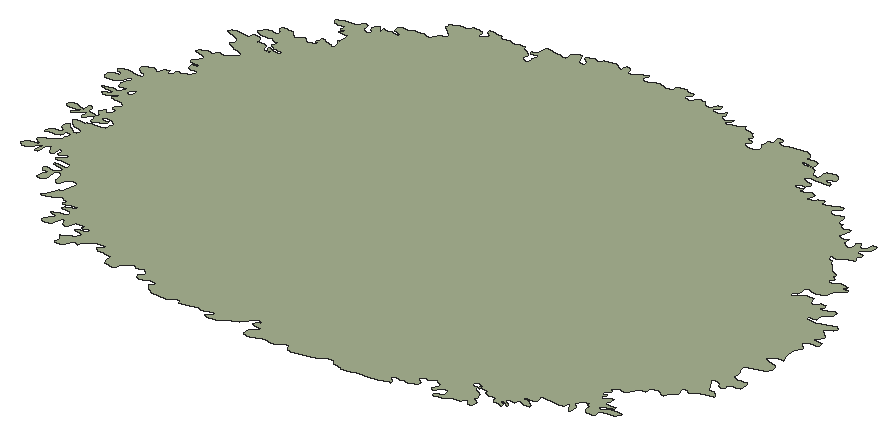
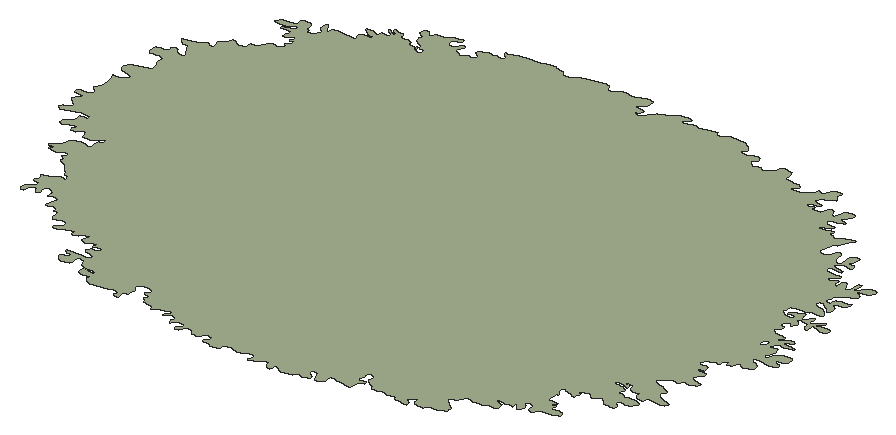
# SketchUp Ruby script. Lengths in inches.
U = 1.inch
M = Sketchup.active_model
def pt(a) = Geom::Point3d.new(a.map { |v| v * U })
def face(e, loops, mat)
  f = e.add_face(loops[0].map { |a| pt(a) })
  loops[1..].each { |l| e.add_face(l.map { |a| pt(a) }).erase! }
  f.material = f.back_material = mat if mat
  f
end
# faces: each face lists its corners as indices into pts; further lists are holes
def faces(e, pts, list, mat = nil) = list.each { |f| face(e, (f[0].is_a?(Array) ? f : [f]).map { |l| l.map { |i| pts[i] } }, mat) }
# xy, xz, yz: faces in a plane at the given z, y or x. An outline is a flat list of corners, or four numbers for a rectangle; further outlines are holes
def ring(l) = l.size == 4 ? [[l[0], l[1]], [l[2], l[1]], [l[2], l[3]], [l[0], l[3]]] : l.each_slice(2).to_a
def flat(e, list, mat, &to3) = list.each { |f| face(e, (f[0].is_a?(Array) ? f : [f]).map { |l| ring(l).map { |u, v| to3.(u, v) } }, mat) }
def xy(e, z, list, mat = nil) = flat(e, list, mat) { |x, y| [x, y, z] }
def xz(e, y, list, mat = nil) = flat(e, list, mat) { |x, z| [x, y, z] }
def yz(e, x, list, mat = nil) = flat(e, list, mat) { |y, z| [x, y, z] }
def lines(e, pts, list) = list.each { |a, b| e.add_line(pt(pts[a]), pt(pts[b])) }
# prism: a flat outline (further loops are holes) pulled along v
def prism(e, loops, v, mat = nil)
  f = face(e, loops, mat); d = Geom::Vector3d.new(v.map { |x| x * U })
  f.pushpull(f.normal.samedirection?(d) ? d.length : -d.length)
end
def box(e, o, s, mat = nil) = prism(e, [[o, [o[0] + s[0], o[1], o[2]], [o[0] + s[0], o[1] + s[1], o[2]], [o[0], o[1] + s[1], o[2]]]], [0, 0, s[2]], mat)
def at(x, y, z, deg = 0) = Geom::Transformation.translation(pt([x, y, z])) * Geom::Transformation.rotation(ORIGIN, Z_AXIS, deg.degrees)
def axes(o, x, y, z) = Geom::Transformation.new([*x, 0, *y, 0, *z, 0, *pt(o).to_a, 1])
def part(name) = M.definitions.add(name)
# library, detail: a bought-in or finely detailed component or shape, given as its bounding box
def library(name, o, s) = part(name).tap { |d| box(d.entities, o, s) }
def detail(e, o, s) = box(e.add_group.entities, o, s)
def put(e, d, t, mat = nil) = e.add_instance(d, t).tap { |i| i.material = mat if mat }
def group(e, t, mat = nil) = e.add_group.tap { |g| g.transformation = t; g.material = mat if mat }.entities
root = M.entities
M.materials.add("Boxwoodplan").color = [166, 177, 144]
xy(root,9.033,[[[36.005,64.445,35.894,64.449,35.799,64.474,35.743,64.53,35.741,64.633,35.768,64.697,35.831,64.76,35.88,64.824,35.938,64.921,35.752,64.951,35.662,64.96,35.682,65.048,35.768,65.106,35.799,65.116,35.794,65.161,35.705,65.193,35.589,65.152,35.492,65.022,35.349,64.867,35.189,64.78,35.083,64.757,35.023,64.732,35.006,64.689,34.862,64.597,34.668,64.567,34.58,64.575,34.499,64.622,34.499,64.643,34.544,64.674,34.635,64.752,34.703,64.799,34.614,64.813,34.502,64.796,34.382,64.751,34.285,64.76,34.188,64.77,34.091,64.762,33.964,64.718,33.764,64.672,33.675,64.665,33.637,64.758,33.629,64.78,33.562,64.788,33.473,64.77,33.304,64.652,33.105,64.643,32.874,64.669,32.707,64.762,32.566,64.926,32.749,65.018,32.649,65.071,32.514,65.088,32.387,65.065,32.315,65.012,32.234,64.988,32.118,65.053,32.077,65.121,32.164,65.162,32.191,65.223,32.195,65.273,32.155,65.325,32.082,65.401,31.997,65.433,31.909,65.38,31.843,65.354,31.787,65.396,31.77,65.419,31.746,65.437,31.717,65.427,31.638,65.373,31.566,65.325,31.49,65.239,31.478,65.106,31.407,65.064,31.357,65.039,31.297,65.041,31.198,65.061,31.111,65.109,31.068,65.177,31.059,65.267,31.068,65.334,31.081,65.355,31.062,65.396,30.849,65.415,30.916,65.451,30.89,65.452,30.798,65.446,30.628,65.462,30.551,65.488,30.533,65.522,30.548,65.54,30.673,65.63,30.671,65.687,30.586,65.709,30.427,65.706,30.297,65.635,30.199,65.549,30.124,65.514,30.077,65.488,30.076,65.469,30.112,65.417,30.096,65.362,30.026,65.397,29.963,65.436,29.901,65.388,29.879,65.333,29.848,65.219,29.8,65.171,29.727,65.137,29.636,65.132,29.566,65.157,29.548,65.19,29.555,65.208,29.576,65.248,29.597,65.307,29.567,65.364,29.465,65.465,29.58,65.545,29.64,65.585,29.72,65.6,29.787,65.631,29.843,65.685,29.927,65.792,29.855,65.818,29.776,65.826,29.644,65.846,29.605,65.881,29.612,65.9,29.687,65.936,29.849,65.973,29.891,66.024,29.887,66.064,29.86,66.079,29.711,66.027,29.665,66.048,29.665,66.067,29.688,66.13,29.527,66.141,29.446,66.149,29.392,66.141,29.385,66.122,29.369,66.025,29.354,65.958,29.3125,65.907,29.266,65.894,29.246,65.909,29.187,65.955,29.143,66.073,29.103,66.099,29.076,66.1,29.022,66.092,29.015,66.073,29.014,65.957,28.959,65.839,28.898,65.765,28.819,65.735,28.739,65.738,28.693,65.763,28.66,65.822,28.66,65.879,28.714,65.993,28.828,66.1,28.848,66.119,28.835,66.139,28.808,66.144,28.728,66.162,28.647,66.175,28.62,66.191,28.627,66.21,28.647,66.229,28.796,66.297,28.958,66.321,29,66.424,28.974,66.485,28.926,66.506,28.899,66.502,28.736,66.484,28.695,66.515,28.702,66.535,28.73,66.595,28.887,66.649,29.059,66.719,29.108,66.758,29.094,66.779,28.998,66.752,28.826,66.733,28.682,66.6875,28.593,66.701,28.566,66.707,28.573,66.727,28.593,66.742,28.648,66.786,28.621,66.823,28.593,66.819,28.511,66.827,28.455,66.875,28.441,66.917,28.414,66.913,28.331,66.89,28.174,66.804,28.025,66.728,27.951,66.696,27.896,66.708,27.909,66.728,27.929,66.768,27.955,66.785,27.979,66.865,28.029,66.966,28.061,67.074,28.112,67.128,28.186,67.167,28.229,67.288,28.251,67.428,28.271,67.542,28.267,67.601,28.222,67.637,28.142,67.65,28.055,67.65,27.981,67.626,27.972,67.561,27.972,67.5,27.939,67.44,27.851,67.403,27.795,67.412,27.756,67.471,27.745,67.532,27.72,67.653,27.714,67.715,27.674,67.769,27.646,67.791,27.608,67.807,27.55,67.795,27.515,67.775,27.513,67.744,27.505,67.682,27.508,67.545,27.533,67.483,27.525,67.419,27.474,67.354,27.426,67.326,27.388,67.314,27.35,67.319,27.308,67.327,27.291,67.354,27.286,67.482,27.308,67.539,27.353,67.592,27.368,67.622,27.36,67.65,27.303,67.655,27.222,67.662,27.184,67.677,27.161,67.706,27.158,67.768,27.174,67.799,27.208,67.815,27.381,67.787,27.459,67.8125,27.509,67.842,27.569,67.889,27.582,67.952,27.559,67.978,27.516,67.979,27.438,67.986,27.346,67.997,27.245,68.033,27.227,68.062,27.232,68.076,27.252,68.079,27.311,68.091,27.486,68.077,27.576,68.102,27.589,68.16,27.5625,68.222,27.49,68.262,27.412,68.268,27.298,68.262,27.198,68.236,27.115,68.254,27.111,68.284,27.132,68.312,27.178,68.369,27.245,68.426,27.298,68.506,27.289,68.54,27.244,68.557,27.179,68.556,27.062,68.455,27.022,68.457,26.987,68.477,27.009,68.536,27.025,68.603,26.982,68.665,26.942,68.682,26.922,68.683,26.916,68.668,26.921,68.622,26.918,68.48,26.877,68.418,26.837,68.423,26.803,68.447,26.705,68.578,26.68,68.643,26.655,68.67,26.64,68.66,26.585,68.609,26.55,68.55,26.569,68.419,26.574,68.352,26.554,68.287,26.505,68.278,26.47,68.294,26.46,68.338,26.48,68.471,26.49,68.549,26.49,68.586,26.475,68.598,26.46,68.587,26.38,68.553,26.34,68.498,26.331,68.435,26.292,68.393,26.155,68.303,26.116,68.293,26.071,68.302,25.991,68.342,25.971,68.372,25.975,68.405,26.008,68.467,26.106,68.552,26.195,68.579,26.285,68.579,26.38,68.583,26.319,68.634,26.168,68.72,26.152,68.781,26.204,68.819,26.296,68.889,26.415,68.951,26.534,69.025,26.569,69.038,26.595,69.062,26.622,69.105,26.625,69.198,26.657,69.318,26.658,69.38,26.637,69.401,26.616,69.41,26.552,69.425,26.519,69.42,26.515,69.404,26.527,69.311,26.486,69.25,26.4375,69.215,26.36,69.186,26.289,69.174,26.129,69.149,26.094,69.154,26.08,69.168,26.08,69.176,26.089,69.216,26.106,69.263,26.148,69.31,26.218,69.357,26.276,69.379,26.334,69.381,26.373,69.383,26.393,69.391,26.416,69.412,26.411,69.436,26.357,69.467,26.289,69.523,26.257,69.58,26.253,69.647,26.266,69.697,26.318,69.742,26.344,69.747,26.356,69.741,26.375,69.727,26.418,69.666,26.467,69.62,26.595,69.542,26.669,69.508,26.704,69.492,26.724,69.5,26.748,69.522,26.755,69.538,26.767,69.579,26.751,69.636,26.709,69.682,26.676,69.705,26.642,69.717,26.583,69.717,26.509,69.72,26.465,69.762,26.379,69.834,26.32,69.885,26.281,69.932,26.282,69.961,26.306,69.987,26.362,70.014,26.398,70.019,26.438,70.015,26.499,69.995,26.56,69.993,26.596,70,26.63,70.041,26.679,70.073,26.739,70.08,26.81,70.079,26.963,70.087,27.104,70.107,27.136,70.124,27.137,70.142,27.131,70.184,27.119,70.228,27.131,70.272,27.16,70.376,27.147,70.399,27.125,70.412,27.068,70.442,27.014,70.479,26.942,70.508,26.868,70.51,26.818,70.5,26.797,70.486,26.772,70.434,26.777,70.413,26.789,70.409,26.812,70.404,26.963,70.392,26.989,70.387,26.994,70.378,26.985,70.362,26.945,70.322,26.9,70.279,26.835,70.243,26.774,70.2,26.701,70.165,26.664,70.168,26.644,70.179,26.619,70.216,26.612,70.311,26.595,70.336,26.613,70.35,26.619,70.393,26.614,70.403,26.602,70.404,26.588,70.402,26.561,70.399,26.529,70.392,26.512,70.38,26.43,70.285,26.399,70.23,26.367,70.207,26.344,70.21,26.318,70.231,26.31,70.248,26.304,70.288,26.332,70.373,26.337,70.418,26.328,70.445,26.308,70.452,26.27,70.444,26.25,70.43,26.204,70.38,26.083,70.273,26.046,70.248,26.021,70.243,25.983,70.25,25.971,70.267,26.0625,70.373,26.125,70.418,26.139,70.444,26.139,70.461,26.13,70.468,26.118,70.464,26.104,70.458,26.072,70.447,25.988,70.423,25.821,70.405,25.748,70.412,25.7,70.437,25.678,70.464,25.677,70.481,25.695,70.533,25.742,70.579,25.803,70.596,25.873,70.6,25.947,70.582,26.075,70.539,26.161,70.513,26.173,70.516,26.172,70.525,26.172,70.535,26.163,70.555,26.138,70.602,26.137,70.658,26.145,70.723,26.156,70.753,26.174,70.765,26.222,70.728,26.261,70.679,26.289,70.633,26.298,70.571,26.31,70.519,26.325,70.492,26.349,70.491,26.483,70.473,26.556,70.46,26.591,70.456,26.609,70.47,26.624,70.518,26.569,70.56,26.511,70.624,26.493,70.651,26.493,70.668,26.527,70.776,26.557,70.799,26.584,70.804,26.599,70.793,26.608,70.775,26.637,70.73,26.649,70.705,26.661,70.707,26.682,70.719,26.762,70.797,26.778,70.843,26.78,70.895,26.765,70.927,26.744,70.939,26.681,70.962,26.642,70.981,26.633,71.002,26.649,71.052,26.705,71.089,26.74,71.111,26.752,71.131,26.76,71.185,26.758,71.232,26.663,71.307,26.519,71.33,26.457,71.346,26.422,71.329,26.394,71.33,26.325,71.347,26.306,71.374,26.315,71.398,26.441,71.5,26.435,71.533,26.413,71.548,26.368,71.54,26.34,71.531,26.214,71.47,26.173,71.423,26.124,71.379,26.055,71.364,26.027,71.366,25.98,71.417,26.008,71.442,26.026,71.481,26.057,71.504,26.151,71.535,26.196,71.565,26.185,71.596,26.172,71.599,26.163,71.592,26.136,71.585,26.097,71.588,25.962,71.6,25.816,71.628,25.792,71.643,25.797,71.662,25.822,71.691,26.035,71.751,26.099,71.75,26.159,71.734,26.22,71.707,26.246,71.709,26.253,71.718,26.302,71.796,26.325,71.811,26.332,71.83,26.331,71.873,26.331,71.898,26.321,71.909,26.307,71.906,26.25,71.907,26.192,71.9,26.145,71.884,26.121,71.891,26.1,71.912,26.075,71.945,26.055,72.033,26.066,72.122,26.096,72.164,26.102,72.196,26.115,72.239,26.153,72.26,26.148,72.306,26.126,72.342,26.037,72.319,26.02,72.285,26.021,72.265,26.024,72.202,25.943,72.155,25.802,72.061,25.647,72.016,25.5625,72.041,25.521,72.094,25.511,72.22,25.64,72.305,25.722,72.319,25.766,72.343,25.789,72.377,25.788,72.397,25.702,72.428,25.629,72.454,25.567,72.51,25.602,72.564,25.679,72.593,25.774,72.627,25.84,72.626,26.018,72.583,26.11,72.562,26.195,72.565,26.246,72.585,26.252,72.605,26.236,72.671,26.175,72.723,26.13,72.73,26.019,72.801,25.972,72.843,25.957,72.879,25.95,72.933,25.951,72.96,25.963,72.975,26.005,73.01,26.056,73.025,26.171,73.056,26.201,73.066,26.242,73.066,26.292,73.061,26.304,73.049,26.319,73.019,26.334,73.005,26.343,73.005,26.371,73.008,26.388,73.02,26.408,73.07,26.436,73.103,26.453,73.126,26.455,73.151,26.471,73.176,26.491,73.188,26.539,73.2,26.578,73.192,26.599,73.149,26.604,73.097,26.62,73.07,26.642,73.07,26.683,73.112,26.708,73.154,26.723,73.258,26.738,73.283,26.77,73.29,26.802,73.29,26.821,73.278,26.843,73.256,26.874,73.255,26.927,73.277,26.971,73.323,26.985,73.347,26.975,73.361,27.034,73.359,27.063,73.362,27.079,73.381,27.084,73.43,27.118,73.47,27.152,73.516,27.099,73.559,27.031,73.588,26.994,73.587,26.961,73.577,26.919,73.565,26.877,73.571,26.856,73.587,26.834,73.61,26.811,73.713,26.824,73.738,26.83,73.755,26.84,73.758,26.944,73.779,26.99,73.787,27.008,73.798,26.998,73.802,26.913,73.83,26.847,73.842,26.818,73.835,26.783,73.835,26.747,73.836,26.711,73.848,26.673,73.898,26.655,73.927,26.655,73.958,26.671,73.979,26.699,73.994,26.731,74.013,26.739,74.041,26.768,74.098,26.795,74.152,26.802,74.205,26.794,74.232,26.754,74.243,26.676,74.27,26.503,74.316,26.467,74.334,26.45,74.358,26.486,74.412,26.531,74.447,26.576,74.474,26.631,74.494,26.683,74.503,26.736,74.5,26.791,74.476,26.847,74.478,26.873,74.482,26.886,74.503,26.904,74.544,26.941,74.58,26.961,74.598,26.988,74.6,27.056,74.583,27.118,74.572,27.145,74.569,27.169,74.584,27.255,74.651,27.342,74.717,27.396,74.814,27.393,74.858,27.351,74.894,27.234,74.932,27.109,74.963,27.022,75.035,26.964,75.07,26.896,75.091,26.868,75.103,26.855,75.124,26.876,75.17,26.925,75.212,26.923,75.297,26.873,75.375,26.742,75.432,26.454,75.528,26.433,75.562,26.505,75.626,26.626,75.678,26.732,75.682,26.788,75.669,26.833,75.643,26.881,75.633,26.934,75.641,26.995,75.653,27.024,75.684,27.039,75.763,27.056,75.798,27.11,75.797,27.167,75.787,27.215,75.767,27.282,75.708,27.307,75.674,27.321,75.634,27.322,75.565,27.328,75.56,27.336,75.565,27.363,75.578,27.414,75.584,27.503,75.586,27.583,75.55,27.617,75.486,27.642,75.408,27.712,75.363,27.752,75.35,27.77,75.35,27.797,75.359,27.893,75.365,27.909,75.371,27.889,75.387,27.826,75.411,27.774,75.415,27.736,75.433,27.717,75.468,27.714,75.48,27.718,75.5,27.733,75.507,27.767,75.507,27.809,75.5,27.915,75.472,28.03,75.467,28.082,75.475,28.101,75.477,28.127,75.489,28.082,75.519,28.041,75.529,27.955,75.544,27.897,75.557,27.856,75.56,27.834,75.564,27.809,75.578,27.758,75.605,27.71,75.631,27.688,75.663,27.699,75.72,27.727,75.758,27.768,75.787,27.728,75.818,27.673,75.833,27.63,75.836,27.575,75.844,27.544,75.87,27.527,75.907,27.512,75.916,27.483,75.915,27.368,75.887,27.316,75.873,27.266,75.874,27.219,75.877,27.169,75.894,27.121,75.911,27.081,75.918,27.038,75.942,26.995,75.965,27.021,75.978,27.022,75.985,27.033,76.025,27.049,76.061,27.075,76.098,27.106,76.13,27.15,76.155,27.203,76.177,27.248,76.189,27.354,76.183,27.431,76.177,27.465,76.173,27.475,76.173,27.475,76.186,27.467,76.228,27.446,76.272,27.41,76.311,27.367,76.342,27.335,76.388,27.336,76.412,27.347,76.432,27.394,76.462,27.447,76.485,27.473,76.485,27.499,76.479,27.554,76.463,27.621,76.458,27.669,76.443,27.692,76.43,27.711,76.411,27.754,76.37,27.793,76.336,27.838,76.304,27.895,76.291,27.948,76.296,27.994,76.325,28.025,76.361,28.074,76.399,28.1,76.399,28.122,76.384,28.163,76.343,28.21,76.309,28.338,76.335,28.412,76.353,28.454,76.381,28.459,76.401,28.438,76.417,28.387,76.439,28.377,76.462,28.385,76.485,28.401,76.529,28.408,76.589,28.412,76.614,28.435,76.631,28.462,76.632,28.493,76.623,28.534,76.604,28.668,76.564,28.729,76.542,28.768,76.509,28.795,76.469,28.81,76.446,28.817,76.438,28.827,76.442,28.834,76.447,28.867,76.492,28.873,76.527,28.863,76.63,28.842,76.678,28.817,76.713,28.782,76.752,28.772,76.781,28.784,76.793,28.795,76.79,28.816,76.792,28.815,76.8,28.82,76.823,28.813,76.865,28.798,77.021,28.8,77.098,28.685,77.117,28.588,77.12,28.526,77.128,28.508,77.135,28.494,77.145,28.507,77.155,28.62,77.197,28.654,77.226,28.654,77.239,28.63,77.263,28.594,77.268,28.542,77.256,28.494,77.234,28.476,77.234,28.461,77.261,28.488,77.344,28.49,77.384,28.489,77.398,28.466,77.419,28.376,77.401,28.264,77.404,28.154,77.42,28.093,77.501,28.091,77.528,28.129,77.565,28.225,77.619,28.274,77.646,28.329,77.651,28.453,77.648,28.545,77.652,28.604,77.661,28.644,77.699,28.684,77.734,28.692,77.777,28.718,77.816,28.774,77.829,28.812,77.824,28.854,77.791,28.866,77.704,28.872,77.616,28.896,77.573,28.952,77.547,29.043,77.527,29.098,77.55,29.116,77.592,29.093,77.634,29.046,77.671,28.99,77.758,29.026,77.837,29.101,77.919,29.119,77.922,29.143,77.892,29.162,77.844,29.236,77.762,29.264,77.736,29.255,77.791,29.237,77.886,29.293,77.903,29.355,77.897,29.481,77.894,29.594,77.891,29.716,77.873,29.735,77.873,29.722,77.902,29.672,77.944,29.541,77.996,29.503,78.005,29.48,78.05,29.483,78.141,29.517,78.186,29.566,78.212,29.682,78.217,29.779,78.226,29.874,78.293,30.001,78.298,30.116,78.287,30.212,78.268,30.333,78.261,30.376,78.307,30.39,78.354,30.433,78.448,30.522,78.502,30.641,78.56,30.653,78.576,30.637,78.609,30.596,78.647,30.489,78.729,30.42,78.802,30.363,78.844,30.305,78.886,30.336,78.893,30.335,78.907,30.33,78.927,30.319,78.995,30.322,79.025,30.358,79.06,30.44,79.1,30.523,79.137,30.561,79.143,30.618,79.141,30.704,79.132,30.728,79.124,30.751,79.126,30.783,79.159,30.835,79.234,30.871,79.248,30.928,79.251,31.03,79.246,31.126,79.214,31.158,79.193,31.1875,79.151,31.189,79.08,31.191,79.052,31.196,79.03,31.219,79.02,31.272,79.031,31.318,79.06,31.379,79.114,31.404,79.138,31.425,79.149,31.438,79.166,31.354,79.213,31.315,79.229,31.272,79.272,31.247,79.351,31.248,79.382,31.307,79.399,31.498,79.37,31.595,79.355,31.631,79.341,31.63,79.295,31.64,79.267,31.7,79.263,31.805,79.278,31.906,79.291,31.948,79.287,31.995,79.273,32.023,79.25,32.047,79.249,32.072,79.258,32.216,79.287,32.257,79.296,32.31,79.303,32.346,79.299,32.39,79.273,32.42,79.202,32.447,79.179,32.491,79.16,32.531,79.149,32.572,79.124,32.623,79.069,32.677,79.012,32.664,78.935,32.658,78.861,32.672,78.831,32.703,78.8,32.729,78.777,32.776,78.769,32.813,78.766,32.857,78.796,32.87,78.828,32.871,78.869,32.859,78.944,32.896,79.103,32.885,79.132,32.867,79.145,32.844,79.148,32.805,79.149,32.752,79.143,32.716,79.142,32.67,79.15,32.644,79.173,32.652,79.195,32.679,79.212,32.718,79.226,32.763,79.253,32.789,79.328,32.792,79.493,32.793,79.525,32.815,79.544,32.841,79.548,32.94,79.538,33.139,79.516,33.231,79.506,33.319,79.485,33.406,79.469,33.457,79.462,33.452,79.67,33.521,79.742,33.605,79.802,33.659,79.792,33.687,79.757,33.736,79.686,33.758,79.612,33.767,79.576,33.764,79.557,33.792,79.522,33.896,79.489,33.948,79.489,33.987,79.52,33.99,79.595,33.888,79.675,33.809,79.734,33.821,79.769,33.865,79.805,33.959,79.856,34.009,79.865,34.09,79.853,34.194,79.853,34.217,79.931,34.427,79.959,34.528,79.977,34.635,79.963,34.714,79.894,34.747,79.859,34.774,79.856,34.814,79.884,34.812,79.959,34.803,80.001,34.816,80.035,34.867,80.045,34.922,80.03,34.992,79.937,35.014,79.863,35.046,79.828,35.095,79.814,35.146,79.818,35.193,79.846,35.281,79.929,35.361,79.983,35.463,80.03,35.512,80.015,35.525,79.979,35.473,79.908,35.447,79.873,35.455,79.831,35.544,79.773,35.644,79.758,35.694,79.767,35.744,79.814,35.823,79.882,35.937,79.897,36.052,79.869,36.083,79.839,36.16,79.808,36.261,79.826,36.342,79.88,36.342,79.993,36.4,80.036,36.513,80.06,36.617,80.055,36.699,79.996,36.845,79.976,36.898,79.967,36.904,79.929,36.831,79.862,36.797,79.789,36.81,79.753,36.881,79.712,36.983,79.716,37.036,79.749,37.056,79.788,37.077,79.86,37.125,79.883,37.149,79.894,37.201,79.894,37.303,79.856,37.347,79.785,37.432,79.732,37.563,79.762,37.597,79.793,37.603,79.836,37.643,79.919,37.75,79.9375,37.78,79.907,37.786,79.866,37.734,79.782,37.685,79.764,37.658,79.729,37.719,79.664,37.849,79.652,37.94,79.688,38.007,79.759,38.032,79.766,38.041,79.748,38.059,79.708,38.084,79.673,38.072,79.616,38.053,79.573,38.07,79.538,38.159,79.495,38.268,79.5,38.323,79.518,38.373,79.573,38.39,79.589,38.392,79.57,38.379,79.528,38.306,79.448,38.272,79.417,38.284,79.382,38.331,79.363,38.388,79.363,38.485,79.404,38.566,79.461,38.786,79.54,38.808,79.469,38.831,79.439,38.882,79.434,38.998,79.426,39.122,79.4,39.137,79.328,39.16,79.298,39.206,79.28,39.229,79.245,39.215,79.208,39.188,79.11,39.305,79.089,39.351,79.07,39.362,79.035,39.288,78.966,39.273,78.929,39.29,78.894,39.365,78.843,39.469,78.816,39.57,78.811,39.682,78.879,39.724,78.954,39.665,79.026,39.633,79.095,39.653,79.201,39.661,79.238,39.632,79.271,39.628,79.307,39.67,79.334,39.771,79.338,39.76,79.4375,39.719,79.59,39.768,79.603,39.833,79.59,39.886,79.572,39.917,79.515,39.867,79.447,39.871,79.411,39.917,79.392,40.025,79.392,40.155,79.426,40.663,79.493,40.708,79.484,40.754,79.46,40.801,79.437,40.834,79.413,40.866,79.343,40.848,79.251,41.053,79.265,41.118,79.258,41.202,79.227,41.239,79.121,41.225,79.073,41.208,79.04,41.167,79.033,40.998,79.064,40.933,79.07,40.89,79.071,40.87,79.065,40.867,79.049,40.896,79.001,40.936,78.981,40.984,78.982,41.156,78.997,41.225,78.999,41.309,78.964,41.347,78.924,41.377,78.862,41.445,78.752,41.524,78.714,41.609,78.709,41.64,78.75,41.634,78.834,41.616,78.886,41.623,78.952,41.664,79.002,41.765,79.034,41.875,79.048,41.963,79.017,42.011,78.975,42.045,78.912,42.046,78.866,41.984,78.811,41.918,78.798,41.877,78.786,41.845,78.753,41.849,78.723,41.899,78.704,41.996,78.679,42.068,78.654,42.087,78.622,42.076,78.591,42.022,78.563,41.934,78.555,41.772,78.549,41.685,78.538,41.597,78.571,41.532,78.585,41.451,78.566,41.394,78.523,41.393,78.459,41.451,78.419,41.537,78.396,41.623,78.381,41.67,78.382,41.704,78.362,41.725,78.319,41.708,78.254,41.673,78.206,41.646,78.181,41.6,78.17,41.458,78.15,41.438,78.145,41.435,78.129,41.429,78.099,41.434,78.066,41.478,78.048,41.545,78.046,41.587,78.046,41.636,78.062,41.699,78.093,41.713,78.028,41.684,77.981,41.678,77.951,41.716,77.932,41.777,77.9375,41.859,77.985,41.915,78.027,41.943,78.052,41.981,78.036,42.045,78.02,42.114,77.967,42.11,77.919,42.067,77.853,42.034,77.788,42.053,77.764,42.099,77.761,42.175,77.771,42.257,77.811,42.296,77.869,42.368,77.912,42.428,77.925,42.465,77.917,42.483,77.893,42.487,77.864,42.469,77.837,42.442,77.8125,42.443,77.798,42.464,77.796,42.636,77.815,42.717,77.826,42.784,77.868,42.826,77.905,42.905,77.93,43.002,77.935,43.025,77.911,43.028,77.882,42.868,77.665,42.883,77.619,42.94,77.567,43.023,77.552,43.112,77.571,43.181,77.599,43.265,77.62,43.33,77.529,43.367,77.315,43.368,77.301,43.404,77.29,43.488,77.311,43.499,77.234,43.523,77.186,43.599,77.177,43.736,77.211,43.804,77.209,43.819,77.155,43.751,76.934,43.74,76.883,43.763,76.83,43.83,76.801,43.897,76.812,44.033,76.839,44.054,76.734,44.049,76.632,44.171,76.563,44.303,76.532,44.334,76.633,44.323,76.737,44.301,76.789,44.329,76.84,44.397,76.851,44.436,76.797,44.458,76.745,44.506,76.71,44.583,76.733,44.637,76.783,44.662,76.899,44.665,76.951,44.726,76.975,44.783,76.947,44.814,76.893,44.788,76.771,44.673,76.691,44.62,76.654,44.6,76.597,44.58,76.547,44.602,76.501,44.734,76.477,44.79,76.449,44.795,76.398,44.722,76.3125,44.757,76.211,44.786,76.159,44.774,76.11,44.64,76.084,44.539,76.044,44.436,75.974,44.384,75.939,44.319,75.942,44.255,75.975,44.222,75.982,44.196,75.959,44.24,75.865,44.359,75.799,44.406,75.76,44.403,75.712,44.488,75.635,44.654,75.448,44.786,75.365,44.85,75.351,44.887,75.308,44.871,75.213,44.987,75.15,44.924,75.064,44.904,75.012,44.902,74.989,44.933,74.976,45.071,74.994,45.205,75.071,45.335,75.084,45.46,75.049,45.464,75.002,45.397,74.976,45.372,74.959,45.385,74.935,45.463,74.915,45.535,74.912,45.567,74.911,45.581,74.887,45.492,74.798,45.326,74.638,45.302,74.547,45.298,74.502,45.27,74.458,45.177,74.383,45.049,74.354,44.924,74.359,44.816,74.398,44.746,74.392,44.719,74.32,44.746,74.21,44.717,74.103,44.599,74.036,44.627,73.936,44.765,73.957,44.937,74.148,45.164,74.131,45.241,73.921,45.285,73.91,45.367,73.934,45.455,74.038,45.593,74.051,45.63,73.951,45.58,73.89,45.566,73.855,45.642,73.816,45.781,73.847,45.901,73.913,45.948,73.929,46.037,73.908,46.015,73.793,45.905,73.699,45.84,73.605,45.847,73.429,45.833,73.394,45.741,73.371,45.608,73.403,45.633,73.297,45.765,73.257,45.91,73.251,46.059,73.281,46.296,73.402,46.432,73.415,46.525,73.323,46.492,73.22,46.351,73.165,46.304,73.141,46.276,73.081,46.379,72.991,46.53,72.831,46.497,72.73,46.381,72.675,46.345,72.651,46.383,72.59,46.527,72.584,46.658,72.5625,46.669,72.461,46.597,72.405,46.463,72.393,46.338,72.356,46.295,72.258,46.463,72.077,46.356,71.884,46.36,71.704,46.414,71.491,46.457,71.393,46.325,71.366,46.202,71.323,46.109,71.247,46.081,71.185,46.192,71.117,46.444,71.06,46.521,70.978,46.542,70.875,46.5,70.783,46.386,70.709,45.924,70.549,45.926,70.457,45.97,70.363,46.024,70.27,46.026,70.179,46.02,70.118,46.017,70.088,46.043,70.034,46.164,69.992,46.289,69.987,46.416,69.997,46.457,69.996,46.515,69.948,46.526,69.769,46.499,69.71,46.39,69.663,46.264,69.645,46.222,69.647,46.176,69.597,46.218,69.507,46.205,69.478,46.12,69.46,46.079,69.461,46.01,69.486,45.977,69.575,45.908,69.607,45.784,69.612,45.742,69.607,45.726,69.548,45.802,69.472,45.889,69.308,45.918,69.285,45.943,69.233,45.961,69.204,46.042,69.193,46.122,69.176,46.207,69.107,46.27,69.026,46.267,68.997,46.183,68.972,45.934,68.931,45.739,68.804,45.666,68.785,45.571,68.86,45.532,68.868,45.468,68.835,45.47,68.75,45.527,68.586,45.484,68.579,45.451,68.535,45.402,68.495,45.348,68.382,45.31,68.334,45.275,68.315,45.239,68.329,45.117,68.416,45.054,68.43,45.012,68.432,44.967,68.413,44.903,68.379,44.873,68.306,44.883,68.253,44.865,68.19,44.703,68.168,44.651,68.126,44.619,68.075,44.572,68.033,44.561,67.971,44.53,67.925,44.495,67.899,44.458,67.888,44.389,67.879,44.291,67.891,44.231,67.866,44.17,67.818,44.14,67.773,44.214,67.735,44.241,67.692,44.205,67.636,44.15,67.6,44.13,67.54,44.128,67.525,44.127,67.51,44.147,67.502,44.218,67.495,44.244,67.498,44.264,67.497,44.268,67.482,44.231,67.412,44.211,67.365,44.208,67.335,44.249,67.334,44.389,67.41,44.457,67.426,44.538,67.423,44.522,67.319,44.505,67.206,44.505,67.158,44.527,67.136,44.568,67.134,44.631,67.161,44.712,67.161,44.771,67.148,44.811,67.143,44.817,67.114,44.777,67.075,44.698,67.046,44.632,67.037,44.549,67.012,44.51,66.974,44.494,66.917,44.497,66.903,44.537,66.902,44.62,66.927,44.777,66.989,44.931,67.019,45.057,67.021,45.11,67.001,45.084,66.927,45.064,66.885,45.002,66.834,44.849,66.808,44.71,66.806,44.65,66.798,44.618,66.743,44.644,66.624,44.629,66.58,44.548,66.559,44.412,66.571,44.354,66.576,44.31,66.63,44.302,66.741,44.301,66.784,44.289,66.812,44.28,66.827,44.261,66.827,44.202,66.84,44.198,66.897,44.199,66.911,44.195,66.926,44.176,66.93,44.096,66.933,44.039,66.907,43.995,66.852,43.957,66.814,43.932,66.756,43.943,66.707,43.999,66.67,44.074,66.57,44.07,66.471,44.061,66.431,44.054,66.404,44.023,66.382,44.004,66.382,43.982,66.413,43.953,66.472,43.888,66.574,43.847,66.613,43.834,66.628,43.823,66.614,43.816,66.587,43.8125,66.543,43.794,66.489,43.788,66.475,43.757,66.459,43.674,66.453,43.533,66.455,43.247,66.456,43.19,66.478,43.103,66.488,43.083,66.479,43.077,66.449,43.128,66.389,43.152,66.291,43.146,66.252,43.114,66.212,43.09,66.205,43.03,66.196,42.927,66.196,42.829,66.2,42.781,66.169,42.837,66.144,42.937,66.129,43.045,66.096,43.12,66.042,43.201,65.97,43.183,65.945,43.122,65.929,43.022,65.937,42.984,65.945,42.934,65.965,42.885,66,42.835,66.024,42.8,65.945,42.79,65.874,42.75,65.861,42.694,65.874,42.65,65.904,42.636,65.916,42.618,65.924,42.606,65.906,42.573,65.829,42.574,65.8,42.608,65.763,42.699,65.732,42.738,65.698,42.751,65.656,42.75,65.642,42.73,65.639,42.687,65.676,42.608,65.725,42.514,65.742,42.457,65.745,42.446,65.731,42.466,65.705,42.581,65.662,42.617,65.651,42.64,65.608,42.637,65.58,42.635,65.566,42.592,65.564,42.479,65.576,42.374,65.611,42.34,65.64,42.331,65.686,42.329,65.757,42.278,65.776,42.219,65.757,42.119,65.765,42.02,65.783,41.994,65.805,41.968,65.842,41.972,65.884,41.978,65.898,41.941,65.907,41.847,65.932,41.808,65.933,41.789,65.934,41.754,65.921,41.742,65.893,41.722,65.887,41.696,65.913,41.692,65.927,41.723,65.951,41.738,65.961,41.73,65.987,41.643,66.044,41.606,66.068,41.587,66.072,41.547,66.052,41.506,66.032,41.487,66.025,41.475,65.997,41.498,65.906,41.594,65.902,41.632,65.897,41.662,65.857,41.655,65.829,41.65,65.815,41.657,65.786,41.769,65.75,41.856,65.712,41.918,65.653,41.934,65.628,41.933,65.614,41.898,65.598,41.878,65.589,41.91,65.567,41.964,65.54,41.976,65.516,41.926,65.483,41.914,65.457,41.939,65.421,42.024,65.377,42.101,65.31,42.1,65.166,42.079,65.141,42.027,65.129,41.973,65.145,41.935,65.189,41.895,65.254,41.877,65.265,41.84,65.26,41.787,65.242,41.766,65.213,41.767,65.169,41.766,65.156,41.732,65.144,41.556,65.134,41.547,65.141,41.499,65.123,41.456,65.092,41.372,65.007,41.319,64.977,41.245,64.967,41.108,64.959,41.054,64.974,41.051,65.013,41.16,65.078,41.261,65.149,41.258,65.252,41.251,65.296,41.252,65.309,41.22,65.331,41.161,65.35,41.086,65.35,41.003,65.266,40.982,65.226,40.925,65.182,40.911,65.173,40.874,65.181,40.838,65.195,40.825,65.222,40.865,65.314,40.925,65.41,40.927,65.451,40.858,65.504,40.747,65.54,40.696,65.562,40.658,65.553,40.634,65.53,40.6,65.487,40.567,65.471,40.524,65.473,40.468,65.482,40.431,65.483,40.393,65.461,40.3125,65.366,40.326,65.325,40.4,65.286,40.455,65.253,40.483,65.232,40.491,65.206,40.468,65.167,40.407,65.123,40.305,65.071,40.25,65.051,40.177,65.054,40.122,65.075,40.049,65.085,40.003,65.06,39.967,65.059,39.934,65.076,39.879,65.081,39.806,65.068,39.784,65.033,39.794,64.975,39.891,64.891,39.919,64.851,39.919,64.813,39.901,64.808,39.611,64.707,39.336,64.685,39.103,64.688,39.012,64.686,38.89,64.625,38.787,64.591,38.69,64.595,38.653,64.596,38.603,64.615,38.555,64.644,38.494,64.641,38.406,64.65,38.321,64.691,38.262,64.748,38.23,64.794,38.172,64.807,38.072,64.794,37.976,64.754,37.896,64.713,37.797,64.64,37.7,64.584,37.607,64.555,37.366,64.537,37.176,64.502,37.08,64.505,37.014,64.6,36.984,64.667,36.895,64.681,36.804,64.668,36.708,64.596,36.643,64.533,36.553,64.526,36.376,64.549,36.191,64.556,36.113,64.505],[26.513,71.73,26.555,71.735,26.575,71.738,26.601,71.746,26.613,71.79,26.614,71.828,26.621,71.913,26.613,71.946,26.601,71.959,26.602,71.973,26.558,71.95,26.502,71.928,26.483,71.922,26.467,71.905,26.445,71.873,26.435,71.836,26.4375,71.791,26.456,71.753,26.475,71.737]]],"Boxwoodplan")
